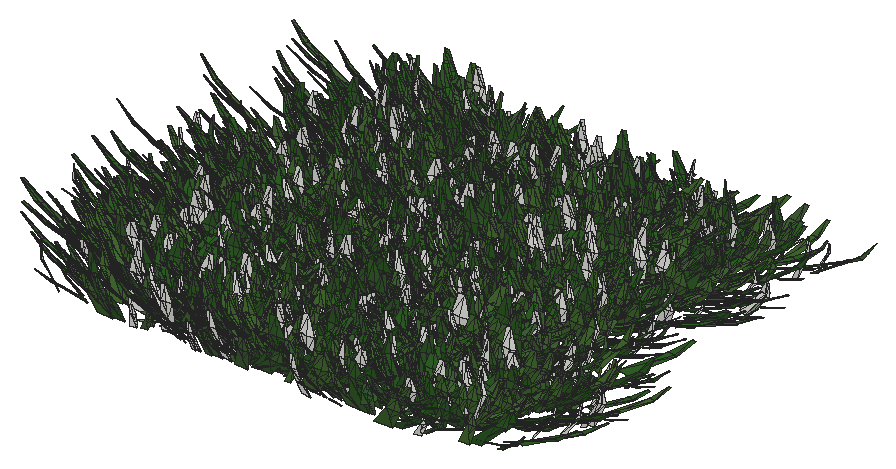
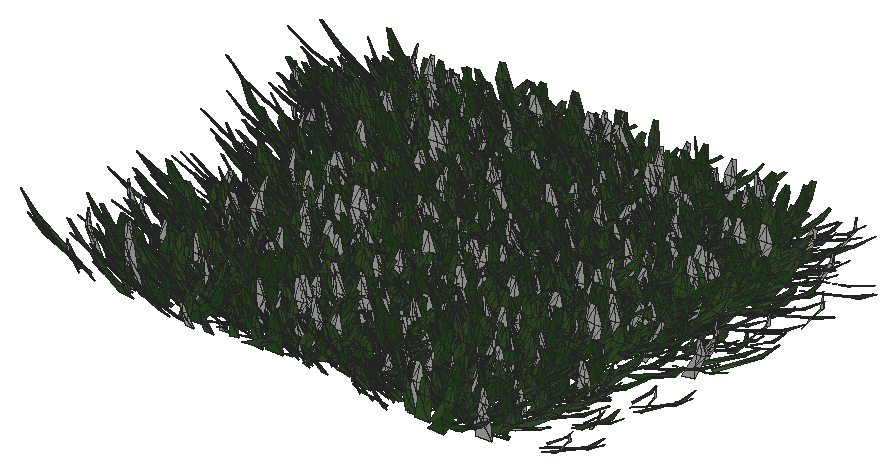
# SketchUp Ruby script. Lengths in inches.
U = 1.inch
M = Sketchup.active_model
def pt(a) = Geom::Point3d.new(a.map { |v| v * U })
def face(e, loops, mat)
  f = e.add_face(loops[0].map { |a| pt(a) })
  loops[1..].each { |l| e.add_face(l.map { |a| pt(a) }).erase! }
  f.material = f.back_material = mat if mat
  f
end
# faces: each face lists its corners as indices into pts; further lists are holes
def faces(e, pts, list, mat = nil) = list.each { |f| face(e, (f[0].is_a?(Array) ? f : [f]).map { |l| l.map { |i| pts[i] } }, mat) }
# xy, xz, yz: faces in a plane at the given z, y or x. An outline is a flat list of corners, or four numbers for a rectangle; further outlines are holes
def ring(l) = l.size == 4 ? [[l[0], l[1]], [l[2], l[1]], [l[2], l[3]], [l[0], l[3]]] : l.each_slice(2).to_a
def flat(e, list, mat, &to3) = list.each { |f| face(e, (f[0].is_a?(Array) ? f : [f]).map { |l| ring(l).map { |u, v| to3.(u, v) } }, mat) }
def xy(e, z, list, mat = nil) = flat(e, list, mat) { |x, y| [x, y, z] }
def xz(e, y, list, mat = nil) = flat(e, list, mat) { |x, z| [x, y, z] }
def yz(e, x, list, mat = nil) = flat(e, list, mat) { |y, z| [x, y, z] }
def lines(e, pts, list) = list.each { |a, b| e.add_line(pt(pts[a]), pt(pts[b])) }
# prism: a flat outline (further loops are holes) pulled along v
def prism(e, loops, v, mat = nil)
  f = face(e, loops, mat); d = Geom::Vector3d.new(v.map { |x| x * U })
  f.pushpull(f.normal.samedirection?(d) ? d.length : -d.length)
end
def box(e, o, s, mat = nil) = prism(e, [[o, [o[0] + s[0], o[1], o[2]], [o[0] + s[0], o[1] + s[1], o[2]], [o[0], o[1] + s[1], o[2]]]], [0, 0, s[2]], mat)
def at(x, y, z, deg = 0) = Geom::Transformation.translation(pt([x, y, z])) * Geom::Transformation.rotation(ORIGIN, Z_AXIS, deg.degrees)
def axes(o, x, y, z) = Geom::Transformation.new([*x, 0, *y, 0, *z, 0, *pt(o).to_a, 1])
def part(name) = M.definitions.add(name)
# library, detail: a bought-in or finely detailed component or shape, given as its bounding box
def library(name, o, s) = part(name).tap { |d| box(d.entities, o, s) }
def detail(e, o, s) = box(e.add_group.entities, o, s)
def put(e, d, t, mat = nil) = e.add_instance(d, t).tap { |i| i.material = mat if mat }
def group(e, t, mat = nil) = e.add_group.tap { |g| g.transformation = t; g.material = mat if mat }.entities
root = M.entities
M.materials.add("Material10").color = [48, 100, 38]
M.materials.add("Material3").color = [68, 110, 58]
M.materials.add("Material4").color = [48, 90, 38]
M.materials.add("Material5").color = [68, 110, 48]
M.materials.add("Material6").color = [48, 90, 48]
M.materials.add("Material7").color = [58, 110, 58]
M.materials.add("Material8").color = [58, 90, 38]
M.materials.add("Material9").color = [68, 100, 58]
c1 = part("grass00")
p = [[-0.6875,0.15,0],[-0.56,0.08,5.52],[-0.04,0.03,2.76],[0.48,-0.02,0],[0.35,-0.02,5.52],[-0.1,-0.14,5.52],
  [-0.12,0.65,8.37],[-0.42,0.65,8.37]]
faces(c1.entities,p,[[0,1,2,3],[3,2,4],[1,5,2],[5,4,2],[1,6,5],[4,5,6],[7,6,1]])
c2 = part("Group16\#1")
put(c2.entities,c1,axes([1.44,-0.61,-0.01],[0.05352,0.12609,0],[-0.10704,0.04543,0.07239],[0.06664,-0.02828,0.11628]),"Material6")
put(c2.entities,c1,axes([0.76,-0.15,-0.01],[0.04676,0.24062,0],[-0.23162,0.04501,0.06642],[0.0652,-0.01267,0.23595]),"Material3")
put(c2.entities,c1,axes([0.79,0.01,-0.01],[-0.00606,0.34651,0],[-0.34381,-0.00602,0.0432],[0.04319,0.00076,0.34386]))
put(c2.entities,c1,axes([1,0.23,-0.01],[-0.07192,0.31144,0],[-0.28722,-0.06632,0.1236],[0.12043,0.02781,0.29478]),"Material5")
put(c2.entities,c1,axes([1.66,0.77,-0.01],[-0.13828,0.29651,0],[-0.21551,-0.1005,0.22471],[0.20365,0.09498,0.23779]),"Material10")
put(c2.entities,c1,axes([0.6875,0.52,-0.01],[-0.18126,0.24051,0],[-0.22746,-0.17142,0.09788],[0.07817,0.05891,0.28481]),"Material5")
put(c2.entities,c1,axes([0.68,0.78,-0.01],[-0.215,0.18688,0],[-0.12385,-0.14248,0.21334],[0.13995,0.16101,0.18878]),"Material3")
put(c2.entities,c1,axes([0.56,1,-0.01],[-0.13756,0.07624,0],[-0.06159,-0.11112,0.0927],[0.04494,0.08108,0.12705]),"Material5")
put(c2.entities,c1,axes([0.2,0.64,-0.01],[-0.23729,0.07254,0],[-0.05711,-0.18681,0.153],[0.04473,0.14632,0.19535]),"Material10")
put(c2.entities,c1,axes([0.0625,0.72,-0.01],[-0.28874,0.02525,0],[-0.02179,-0.24916,0.14647],[0.01276,0.14591,0.25012]),"Material3")
put(c2.entities,c1,axes([-0.08,0.62,-0.01],[-0.34089,-0.04187,0],[0.03255,-0.26504,0.216],[-0.02633,0.21439,0.26703]),"Material10")
put(c2.entities,c1,axes([-0.34,0.98,-0.01],[-0.14314,-0.0493,0],[0.04397,-0.12769,0.06843],[-0.02228,0.0647,0.13505]),"Material10")
put(c2.entities,c1,axes([-0.87,1.45,-0.01],[-0.23488,-0.14114,0],[0.13761,-0.22901,0.06087],[-0.03135,0.05217,0.26717]))
put(c2.entities,c1,axes([-0.72,0.77,-0.01],[-0.14208,-0.13251,0],[0.07209,-0.0773,0.16301],[-0.11118,0.11922,0.1057]),"Material10")
put(c2.entities,c1,axes([-0.62,0.43,-0.01],[-0.14845,-0.21203,0],[0.18654,-0.13061,0.12304],[-0.10079,0.07057,0.22772]),"Material3")
put(c2.entities,c1,axes([-0.68,0.29,-0.01],[-0.13639,-0.32136,0],[0.31723,-0.13464,0.05579],[-0.05136,0.0218,0.34462]),"Material4")
put(c2.entities,c1,axes([-0.64,0.125,-0.01],[-0.0458,-0.23569,0],[0.22124,-0.043,0.08276],[-0.08124,0.01579,0.22538]),"Material7")
put(c2.entities,c1,axes([-1.6,-0.03,-0.01],[0.00576,-0.32897,0],[0.27526,0.00482,0.18018],[-0.18015,-0.00315,0.2753]),"Material5")
put(c2.entities,c1,axes([-1.36,-0.31,-0.01],[0.05718,-0.24765,0],[0.18172,0.04196,0.17267],[-0.16825,-0.03885,0.1865]),"Material10")
put(c2.entities,c1,axes([-1.54,-0.72,-0.01],[0.06537,-0.14017,0],[0.13555,0.06321,0.03939],[-0.0357,-0.01665,0.14956]))
put(c2.entities,c1,axes([-1.19,-0.9,-0.01],[0.09597,-0.12735,0],[0.11214,0.08451,0.07557],[-0.06035,-0.04548,0.14042]),"Material9")
put(c2.entities,c1,axes([-0.47,-0.54,-0.01],[0.11588,-0.10072,0],[0.0618,0.0711,0.12124],[-0.07953,-0.0915,0.0942]))
put(c2.entities,c1,axes([-0.47,-0.84,-0.01],[0.11927,-0.0661,0],[0.06603,0.11913,0.00646],[-0.00313,-0.00565,0.13621]),"Material5")
put(c2.entities,c1,axes([-0.38,-1.24,-0.01],[0.28037,-0.08571,0],[0.0618,0.20215,0.20315],[-0.05939,-0.19428,0.21139]),"Material9")
put(c2.entities,c1,axes([-0.06,-0.66,-0.01],[0.22719,-0.01987,0],[0.01247,0.14255,0.17758],[-0.01547,-0.17691,0.1431]),"Material8")
put(c2.entities,c1,axes([0.11,-0.89,-0.01],[0.14882,0.01828,0],[-0.01058,0.08611,0.12229],[0.01491,-0.12138,0.08676]),"Material6")
put(c2.entities,c1,axes([0.25,-0.72,-0.01],[0.20481,0.07053,0],[-0.06206,0.18022,0.10291],[0.03351,-0.0973,0.1906]),"Material6")
put(c2.entities,c1,axes([0.85,-1.42,-0.01],[0.16481,0.09904,0],[-0.09472,0.15762,0.05616],[0.02893,-0.04814,0.18389]),"Material5")
put(c2.entities,c1,axes([1.01,-1.09,-0.01],[0.21858,0.20385,0],[-0.17495,0.1876,0.15339],[0.10462,-0.11218,0.25652]),"Material10")
put(c2.entities,c1,axes([1.01,-0.71,-0.01],[0.08733,0.12473,0],[-0.06445,0.04512,0.13037],[0.1068,-0.07477,0.07867]),"Material6")
c3 = part("Group15\#1")
put(c3.entities,c2,at(0,0,0))
c4 = part("3darcstudiotree_grass00\#1")
put(c4.entities,c3,at(0,0,0))
put(root,c4,axes([993.08,950.1,0],[-3.70141,-0.8816,0],[3.55908,-0.93393,-0.03405],[0.10659,-0.02797,1.46358]))
put(root,c4,axes([990.92,944.4375,0],[1.53914,1.0513,0],[-4.39566,0.40221,-0.03042],[-0.15696,0.01436,1.60735]))
put(root,c4,axes([991.4,954.42,0],[4.38638,0.43915,0],[-1.65781,1.03492,-0.05201],[-0.12203,0.07618,1.75905]))
put(root,c4,axes([992.45,966.72,0],[3.5333,-0.35922,0],[1.45173,0.89244,-0.02601],[0.05982,0.03677,1.4702]))
put(root,c4,axes([992.18,962.12,0],[4.6185,-0.19049,0],[0.64707,0.98053,-0.03976],[0.0459,0.06956,1.7619]))
put(root,c4,axes([992.69,939.44,0],[-0.10897,1.07036,0],[-4.26555,-0.02714,-0.03168],[-0.19713,-0.00125,1.66016]))
put(root,c4,axes([993.28,951.7,0],[3.42773,-0.49366,0],[2.33187,1.01196,-0.00508],[0.01362,0.00591,1.56982]))
put(root,c4,axes([992.8,948.71,0],[1.88253,1.20428,0],[-4.05103,0.39579,-0.05423],[-0.25457,0.02487,1.37014]))
put(root,c4,axes([994.36,945.55,0],[1.67023,-1.19421,0],[4.03376,0.3526,-0.01723],[0.08743,0.00764,1.43549]))
put(root,c4,axes([993.875,938.22,0],[-2.65738,1.09384,0],[-4.1127,-0.62446,-0.06137],[-0.25477,-0.03868,1.46064]))
put(root,c4,axes([993.53,942.125,0],[3.93411,-0.32217,0],[1.27665,0.97436,-0.03684],[0.07239,0.05525,1.61813]))
put(root,c4,axes([993.77,971.11,0],[4.66298,-0.3319,0],[1.18544,1.04091,-0.0361],[0.05479,0.04811,1.4995]))
put(root,c4,axes([994.79,946.65,0],[-3.31735,0.93033,0],[-2.98242,-0.66466,-0.02096],[-0.10528,-0.02346,1.6805]))
put(root,c4,axes([994.64,957.16,0],[-1.67728,0.97063,0],[-4.3061,-0.46507,-0.05011],[-0.26514,-0.02864,1.6899]))
put(root,c4,axes([995.03,955.6,0],[-2.6954,0.74968,0],[-3.20953,-0.72123,-0.05045],[-0.20663,-0.04643,1.48531]))
put(root,c4,axes([994.5,965.08,0],[0.74763,1.2665,0],[-3.58863,0.1324,-0.00575],[-0.0331,0.00122,1.31904]))
put(root,c4,axes([994.71,933.67,0],[0.50371,0.92792,0],[-3.91618,0.13287,-0.02967],[-0.18729,0.00635,1.57371]))
put(root,c4,axes([996.82,964.2,0],[-3.39734,-0.81214,0],[3.21264,-0.83994,-0.00934],[0.03489,-0.00912,1.57129]))
put(root,c4,axes([994.63,952.85,0],[2.9171,1.0312,0],[-3.90665,0.69071,-0.03132],[-0.15312,0.02707,1.7905]))
put(root,c4,axes([997.03,966.61,0],[-3.12061,-0.47334,0],[2.372,-0.97738,-0.04577],[0.16283,-0.06709,1.96036]))
put(root,c4,axes([997.5625,964.73,0],[-4.51264,-0.18826,0],[0.71719,-1.07444,-0.03361],[0.0313,-0.04689,1.54092]))
put(root,c4,axes([997.93,954.32,0],[-1.81184,-1.16372,0],[3.89157,-0.37868,-0.00938],[0.0544,-0.00529,1.62403]))
put(root,c4,axes([998.05,947.21,0],[-2.30449,-0.91323,0],[3.99186,-0.62958,-0.04882],[0.19366,-0.03054,1.38366]))
put(root,c4,axes([997.91,958.86,0],[-3.97113,-0.2451,0],[1.12308,-1.13729,-0.03453],[0.04096,-0.04148,1.44935]))
put(root,c4,axes([996.7,962.68,0],[0.9039,1.10782,0],[-3.7396,0.1907,-0.03877],[-0.30879,0.01575,1.93915]))
put(root,c4,axes([997.12,943.48,0],[4.31287,-0.5541,0],[2.34742,1.14195,-0.04443],[0.08836,0.04298,1.39643]))
put(root,c4,axes([998.5,949.51,0],[-2.23159,-0.76023,0],[4.05726,-0.74436,-0.05528],[0.25257,-0.04634,1.78248]))
put(root,c4,axes([998.52,948.84,0],[-4.02658,-0.46054,0],[1.58874,-0.86816,-0.02741],[0.08919,-0.04874,1.86713]))
put(root,c4,axes([996.73,951.7,0],[4.23303,0.24806,0],[-0.88984,0.94903,-0.007],[-0.01026,0.01094,1.56436]))
put(root,c4,axes([997.01,956.24,0],[0.42645,1.00239,0],[-4.44972,0.11832,-0.05804],[-0.28832,0.00767,1.39706]))
put(root,c4,axes([997,970.93,0],[3.77106,0.1861,0],[-0.77685,0.98386,-0.02055],[-0.02979,0.03773,1.87683]))
put(root,c4,axes([998.93,940.92,0],[-3.30832,-0.44964,0],[1.76308,-0.81076,-0.02167],[0.05991,-0.02755,1.33527]))
put(root,c4,axes([998.79,960.9375,0],[-4.45965,0.06137,0],[-0.23794,-1.08073,-0.00024],[-0.00009,-0.00042,1.85086]))
put(root,c4,axes([998.5,935.0625,0],[-3.86065,0.46316,0],[-1.72487,-0.89859,-0.02803],[-0.09373,-0.04883,1.92571]))
put(root,c4,axes([997.53,972.55,0],[0.27692,1.06146,0],[-3.97037,0.06474,-0.03468],[-0.23973,0.00391,1.72254]))
put(root,c4,axes([998.02,945.57,0],[4.229,-0.39119,0],[1.33455,0.9017,-0.04569],[0.11742,0.07934,1.78027]))
put(root,c4,axes([999.43,969.71,0],[-4.92673,0.10496,0],[-0.34343,-1.00748,-0.04489],[-0.0281,-0.08244,1.86365]))
put(root,c4,axes([998.88,942.19,0],[2.71553,-0.59411,0],[3.06461,0.87548,-0.0129],[0.0406,0.0116,1.39029]))
put(root,c4,axes([998.58,953.56,0],[4.13058,-0.51477,0],[2.24071,1.12373,-0.00236],[0.00471,0.00236,1.40454]))
put(root,c4,axes([999.89,968.64,0],[-4.32782,-0.07969,0],[0.34618,-1.17501,-0.00991],[0.00419,-0.01422,1.69565]))
put(root,c4,axes([998.53,937.6875,0],[4.87575,-0.07031,0],[0.2378,1.03062,-0.03809],[0.01526,0.06615,1.79573]))
put(root,c4,axes([999,936.71,0],[4.34695,-0.61956,0],[2.03841,0.89387,-0.05304],[0.19031,0.08345,1.86337]))
put(root,c4,axes([1000.55,939.22,0],[-0.06657,-0.97228,0],[3.61389,-0.01547,-0.01279],[0.09363,-0.0004,1.65408]))
put(root,c4,axes([1000.48,957.67,0],[-0.52118,1.08575,0],[-3.57431,-0.10723,-0.01529],[-0.11274,-0.00338,1.67142]))
put(root,c4,axes([1002.68,939.83,0],[-0.33547,-0.93865,0],[4.62281,-0.10326,-0.01785],[0.11677,-0.00261,1.90542]))
put(root,c4,axes([1002.77,940.375,0],[0.01005,-1.20258,0],[4.19815,0.00219,-0.00952],[0.05269,0.00003,1.45276]))
put(root,c4,axes([1003.34,957.1,0],[-4.31518,-0.12187,0],[0.57213,-1.26614,-0.03054],[0.01977,-0.04376,1.83699]))
put(root,c4,axes([1003.46,962.26,0],[-3.97014,0.26009,0],[-1.01896,-0.97211,-0.00505],[-0.00887,-0.00846,1.74136]))
put(root,c4,axes([1002.71,951.42,0],[3.84845,-0.37536,0],[1.314,0.842,-0.03886],[0.09501,0.06088,1.52001]))
put(root,c4,axes([1004.52,971.2,0],[-3.84586,-0.50053,0],[1.98165,-0.95164,-0.02288],[0.06035,-0.02898,1.53217]))
put(root,c4,axes([1004.54,956.28,0],[1.58704,-0.95278,0],[3.80003,0.3956,-0.04485],[0.25602,0.02665,1.59096]))
put(root,c4,axes([1003.58,937.61,0],[0.72703,0.98679,0],[-4.37824,0.20161,-0.0472],[-0.24448,0.01126,1.46547]))
put(root,c4,axes([1003.69,953.25,0],[2.85718,1.03717,0],[-3.15985,0.54404,-0.04649],[-0.2079,0.0358,1.30192]))
put(root,c4,axes([1003.82,945.07,0],[4.19495,0.19536,0],[-0.69064,0.92689,-0.03922],[-0.04451,0.05974,1.46066]))
put(root,c4,axes([1004.42,955.03,0],[3.26699,-0.39523,0],[1.71248,0.88472,-0.0104],[0.02647,0.01367,1.43546]))
put(root,c4,axes([1003.76,963.12,0],[0.48352,1.11677,0],[-5.03625,0.13628,-0.03135],[-0.15085,0.00408,1.53244]))
put(root,c4,axes([1004.44,965.01,0],[4.15736,-0.22719,0],[0.90665,1.03692,-0.02018],[0.02441,0.02792,1.50307]))
put(root,c4,axes([1006.59,948.11,0],[-2.6745,-0.8431,0],[3.5822,-0.71022,-0.01126],[0.04091,-0.00811,1.32461]))
put(root,c4,axes([1006.23,944.43,0],[-3.71389,-0.2193,0],[0.91243,-0.96576,-0.01801],[0.02228,-0.02358,1.33554]))
put(root,c4,axes([1006.1,942.16,0],[-1.37594,-0.94184,0],[3.46555,-0.31643,-0.03784],[0.25579,-0.02336,1.65933]))
put(root,c4,axes([1006.53,967.89,0],[-0.30959,-1.20063,0],[5.07298,-0.08176,-0.03565],[0.17141,-0.00276,1.53082]))
put(root,c4,axes([1006.7,949.87,0],[-5.13737,-0.16678,0],[0.63051,-1.21389,-0.02421],[0.01691,-0.03256,1.66024]))
put(root,c4,axes([1005.71,966.95,0],[2.61832,-0.717,0],[3.31257,0.75605,-0.05494],[0.2657,0.06064,1.83588]))
put(root,c4,axes([1005.74,936.28,0],[4.35597,0.12735,0],[-0.44802,0.95775,-0.0104],[-0.00937,0.02004,1.87036]))
put(root,c4,axes([1006.67,961.1,0],[2.88619,-0.79207,0],[3.8321,0.87272,-0.04921],[0.18723,0.04264,1.66765]))
put(root,c4,axes([1006.53,959.3,0],[-2.47521,0.9479,0],[-4.1372,-0.67521,-0.02867],[-0.13874,-0.02264,1.78429]))
put(root,c4,axes([1006.01,933.64,0],[3.15699,0.44702,0],[-1.9309,0.8523,-0.02459],[-0.09443,0.04168,1.90817]))
put(root,c4,axes([1006.77,947.3,0],[4.16611,-0.6608,0],[2.43007,0.95755,-0.04672],[0.16308,0.06426,1.84728]))
put(root,c4,axes([1006.1,934.39,0],[3.70483,0.88926,0],[-3.42802,0.89261,-0.04664],[-0.18584,0.04839,1.77978]))
put(root,c4,axes([1006.75,969.4,0],[1.28426,1.18436,0],[-4.11752,0.27905,-0.02312],[-0.12583,0.00853,1.50331]))
put(root,c4,axes([1009.34,949.63,0],[2.28346,-0.77469,0],[3.44717,0.63505,-0.04551],[0.22499,0.04145,1.64335]))
put(root,c4,axes([1009.38,945.4,0],[-3.11661,0.81451,0],[-3.35485,-0.80231,-0.01205],[-0.05625,-0.01345,1.87482]))
put(root,c4,axes([1010.51,938.44,0],[-4.56857,-0.03056,0],[0.12408,-1.1593,-0.01377],[0.0021,-0.01961,1.65227]))
put(root,c4,axes([1010.05,955.05,0],[-3.49798,0.58152,0],[-2.29705,-0.86358,-0.00165],[-0.005,-0.00188,1.42237]))
put(root,c4,axes([1011.08,942.18,0],[-3.54461,-0.42652,0],[2.22844,-1.15748,-0.00367],[0.00795,-0.00413,1.60507]))
put(root,c4,axes([1010.65,936.26,0],[0.72449,-1.28293,0],[4.25597,0.15021,-0.01886],[0.1212,0.00428,1.74385]))
put(root,c4,axes([1009.57,952.7,0],[4.06118,0.1391,0],[-0.5324,0.97148,-0.00884],[-0.00926,0.01689,1.89082]))
put(root,c4,axes([1009.73,970.2,0],[3.80962,0.48399,0],[-2.27163,1.11755,-0.02666],[-0.05719,0.02813,1.48409]))
put(root,c4,axes([1010.35,934.4,0],[-1.84818,0.79503,0],[-4.49204,-0.65265,-0.02835],[-0.13063,-0.01898,1.73088]))
put(root,c4,axes([1011.93,965.32,0],[-4.49893,-0.43837,0],[1.53995,-0.98776,-0.03755],[0.08017,-0.05142,1.55797]))
put(root,c4,axes([1010.35,963.24,0],[4.7752,0.14497,0],[-0.46713,0.96169,-0.01966],[-0.01749,0.036,1.78732]))
put(root,c4,axes([1010.83,957.28,0],[-1.92575,0.83965,0],[-4.05155,-0.58077,-0.01882],[-0.10891,-0.01561,1.94745]))
put(root,c4,axes([1012.52,962.59,0],[-1.58063,-0.88051,0],[4.29272,-0.48163,-0.01184],[0.05795,-0.0065,1.57815]))
put(root,c4,axes([1012.26,966.58,0],[-0.4942,-0.9258,0],[4.62783,-0.1544,-0.03174],[0.19168,-0.0064,1.77768]))
put(root,c4,axes([1011.22,940.77,0],[4.19202,-0.62373,0],[2.32182,0.97529,-0.02674],[0.0725,0.03045,1.50406]))
put(root,c4,axes([1012.4,968.29,0],[-2.7199,-1.09643,0],[3.70626,-0.57463,-0.05324],[0.3066,-0.04754,1.84703]))
put(root,c4,axes([1012.27,951.14,0],[-4.05366,0.12739,0],[-0.60907,-1.21134,-0.04842],[-0.03855,-0.07666,1.94818]))
put(root,c4,axes([1011.39,948.84,0],[5.04215,0.13014,0],[-0.5216,1.26309,-0.06196],[-0.03085,0.07472,1.53928]))
put(root,c4,axes([1011.625,939.08,0],[4.01222,0.17516,0],[-0.82819,1.18564,-0.04039],[-0.03228,0.04621,1.39779]))
put(root,c4,axes([1011.9,947.32,0],[3.70391,0.67264,0],[-2.69019,0.92586,-0.05492],[-0.18493,0.06364,1.63919]))
put(root,c4,axes([1013.2,970.81,0],[-3.854,0.71401,0],[-2.71385,-0.91553,-0.03727],[-0.14645,-0.04941,1.88005]))
put(root,c4,axes([1012.6,956.61,0],[3.9405,-0.83524,0],[2.79845,0.82516,-0.04452],[0.20818,0.06139,1.95574]))
put(root,c4,axes([1011.73,959.53,0],[2.7963,0.73348,0],[-3.70563,0.88296,-0.0237],[-0.07242,0.01726,1.35093]))
put(root,c4,axes([1012.88,944.37,0],[3.48051,0.83109,0],[-2.69675,0.70586,-0.00574],[-0.02303,0.00603,1.41814]))
put(root,c4,axes([1013.1,960.93,0],[1.55604,0.87534,0],[-4.29389,0.47706,-0.00487],[-0.02529,0.00281,1.66894]))
put(root,c4,axes([1016.02,936.34,0],[-4.60072,-0.1914,0],[0.66397,-0.99747,-0.03971],[0.03807,-0.05719,1.4765]))
put(root,c4,axes([1015.3,968.43,0],[-2.80563,0.59342,0],[-3.19145,-0.94305,-0.04396],[-0.1676,-0.04953,1.82298]))
put(root,c4,axes([1015.375,969.18,0],[-3.36424,0.91814,0],[-3.26593,-0.74794,-0.02313],[-0.11922,-0.0273,1.93523]))
put(root,c4,axes([1015.37,941.01,0],[3.31986,-0.90832,0],[2.95695,0.67547,-0.04297],[0.18756,0.04285,1.48019]))
put(root,c4,axes([1015.27,942.84,0],[4.45796,-0.3025,0],[1.23547,1.13796,-0.0215],[0.03263,0.03006,1.70776]))
put(root,c4,axes([1015.01,960.45,0],[1.59432,0.97436,0],[-4.70635,0.4813,-0.06498],[-0.3656,0.03739,1.93183]))
put(root,c4,axes([1015.625,950.4,0],[4.36905,-0.5157,0],[1.63569,0.86611,-0.01833],[0.04371,0.02315,1.33779]))
put(root,c4,axes([1015.54,951.82,0],[-2.09066,0.8963,0],[-4.13643,-0.60302,-0.00159],[-0.00743,-0.00108,1.61385]))
put(root,c4,axes([1015.46,964.9,0],[3.77784,0.09096,0],[-0.38847,1.00844,-0.03978],[-0.02973,0.07718,1.9745]))
put(root,c4,axes([1016.16,957.25,0],[4.39293,-0.39638,0],[1.51129,1.04681,-0.00463],[0.01009,0.00699,1.7876]))
put(root,c4,axes([1017.8,935.34,0],[-2.80912,-0.5814,0],[2.98833,-0.9024,-0.02106],[0.0666,-0.02011,1.45262]))
put(root,c4,axes([1015.59,947.99,0],[1.32804,0.89243,0],[-4.56048,0.42416,-0.01219],[-0.04894,0.00455,1.30286]))
put(root,c4,axes([1016.95,943.6,0],[-3.32952,0.73934,0],[-2.566,-0.72222,-0.02123],[-0.07998,-0.02251,1.37003]))
put(root,c4,axes([1017.18,947.54,0],[1.3987,-1.16529,0],[3.94932,0.29627,-0.0465],[0.25173,0.01888,1.45674]))
put(root,c4,axes([1016.17,939.12,0],[4.48384,-0.0442,0],[0.16896,1.07134,-0.03451],[0.00949,0.06019,1.8714]))
put(root,c4,axes([1018.1,971.47,0],[-2.9743,-0.97046,0],[3.84774,-0.73704,-0.04805],[0.20355,-0.03899,1.61679]))
put(root,c4,axes([1016.11,937.74,0],[3.76585,0.33599,0],[-1.61193,1.12919,-0.03925],[-0.05722,0.04008,1.29995]))
put(root,c4,axes([1017.62,966.16,0],[1.03504,-1.15768,0],[4.4608,0.24927,-0.0396],[0.20091,0.01123,1.48525]))
put(root,c4,axes([1017.12,959.42,0],[3.13436,-0.48515,0],[2.36256,0.95397,-0.03178],[0.09873,0.03987,1.65559]))
put(root,c4,axes([1016.8125,963.28,0],[2.27275,0.69978,0],[-3.25332,0.66039,-0.04172],[-0.2207,0.0448,1.78477]))
put(root,c4,axes([1018.49,961.87,0],[0.03995,-0.91638,0],[3.85114,0.01049,-0.01263],[0.08929,0.00024,1.70174]))
put(root,c4,axes([1018.74,945.21,0],[-0.0743,-1.09346,0],[5.15443,-0.02189,-0.0635],[0.38021,-0.00161,1.92948]))
put(root,c4,axes([1018.35,954.79,0],[-0.87822,1.20362,0],[-5.10038,-0.23259,-0.02378],[-0.14141,-0.00645,1.95907]))
put(root,c4,axes([1018.68,933.62,0],[-1.6227,0.88053,0],[-4.355,-0.50161,-0.00587],[-0.0262,-0.00302,1.47291]))
put(root,c4,axes([1018.72,955.59,0],[4.89448,0.02106,0],[-0.07768,1.1284,-0.04862],[-0.00413,0.05993,1.39123]))
put(root,c4,axes([1019.23,952.88,0],[3.93844,-0.46233,0],[1.56764,0.83463,-0.03796],[0.10707,0.05701,1.52986]))
put(root,c4,axes([1021.36,940.96,0],[-4.19523,0.01101,0],[-0.04384,-1.04387,-0.01485],[-0.00097,-0.02314,1.62647]))
put(root,c4,axes([1021.25,960.9,0],[2.74476,-0.63144,0],[3.24378,0.88126,-0.00074],[0.00283,0.00077,1.68668]))
put(root,c4,axes([1021.92,950.5,0],[-1.38491,-0.87134,0],[4.17889,-0.41512,-0.04918],[0.21859,-0.02171,1.34418]))
put(root,c4,axes([1021.29,956.09,0],[-2.83927,0.94701,0],[-3.75848,-0.70428,-0.01976],[-0.09358,-0.01754,1.7373]))
put(root,c4,axes([1021.03,957.5,0],[4.64321,-0.10228,0],[0.43492,1.23399,-0.00682],[0.00288,0.00819,1.49182]))
put(root,c4,axes([1022.4,951.83,0],[0.60172,-0.90687,0],[4.84176,0.20079,-0.06063],[0.30013,0.01245,1.53907]))
put(root,c4,axes([1021.15,966.8,0],[4.59228,0.4506,0],[-1.57539,1.00348,-0.00074],[-0.00157,0.001,1.56313]))
put(root,c4,axes([1023.3,958.86,0],[-4.3908,-0.21331,0],[0.95341,-1.22655,-0.00093],[0.00081,-0.00104,1.42207]))
put(root,c4,axes([1023.45,964.87,0],[-2.23417,-0.72587,0],[3.44566,-0.66284,-0.03027],[0.1304,-0.02509,1.47708]))
put(root,c4,axes([1021.53,954.76,0],[0.72512,1.17526,0],[-3.95245,0.15241,-0.0058],[-0.04155,0.0016,1.813]))
put(root,c4,axes([1023.16,943.56,0],[1.59637,-0.98272,0],[4.08137,0.41437,-0.04502],[0.2819,0.02862,1.86083]))
put(root,c4,axes([1022.8,936.9,0],[3.44919,-0.8389,0],[2.51647,0.64667,-0.01443],[0.08324,0.02139,1.86565]))
put(root,c4,axes([1024.07,946.57,0],[-4.3854,-0.36655,0],[1.15878,-0.86648,-0.00172],[0.00341,-0.00255,1.42531]))
put(root,c4,axes([1024.18,937.46,0],[-1.10015,-1.07569,0],[4.31851,-0.27604,-0.04783],[0.26751,-0.0171,1.6084]))
put(root,c4,axes([1024.53,963.45,0],[-2.44496,-0.90858,0],[3.92777,-0.66059,-0.0439],[0.19033,-0.03201,1.54604]))
put(root,c4,axes([1022.54,953.47,0],[3.01882,0.54467,0],[-2.85178,0.98787,-0.01696],[-0.0599,0.02075,1.8379]))
put(root,c4,axes([1022.78,945.96,0],[1.72651,0.80182,0],[-4.15188,0.55875,-0.00648],[-0.03257,0.00438,1.68262]))
put(root,c4,axes([1024.76,971.45,0],[-4.67562,0.03677,0],[-0.12525,-0.99545,-0.03177],[-0.00796,-0.06328,1.98473]))
put(root,c4,axes([1023,967.87,0],[3.74443,0.79231,0],[-2.92784,0.86481,-0.04954],[-0.20172,0.05958,1.78537]))
put(root,c4,axes([1025.29,938.84,0],[-0.41267,-0.99142,0],[5.06334,-0.13172,-0.00351],[0.0163,-0.00042,1.48465]))
put(root,c4,axes([1023.33,935.42,0],[4.97186,0.0872,0],[-0.33381,1.18949,-0.05051],[-0.02266,0.08074,1.91076]))
put(root,c4,axes([1025.3,969.89,0],[-2.51888,-0.8121,0],[2.88545,-0.55936,-0.0081],[0.05261,-0.0102,1.87526]))
put(root,c4,axes([1024.9,962.09,0],[0.49939,-1.21812,0],[4.94049,0.12659,-0.06373],[0.30684,0.00786,1.50237]))
put(root,c4,axes([1024.86,941.89,0],[1.78182,-0.82345,0],[4.25701,0.57572,-0.03985],[0.17401,0.02353,1.5017]))
put(root,c4,axes([1024.38,948.32,0],[4.57283,0.48925,0],[-2.0405,1.19199,-0.06274],[-0.14636,0.0855,1.92197]))
put(root,c4,axes([1027.01,942.97,0],[-4.16521,-0.5533,0],[2.06422,-0.97121,-0.03648],[0.11162,-0.05251,1.79293]))
put(root,c4,axes([1026.9375,941.37,0],[-2.37661,-1.01523,0],[3.11528,-0.4558,-0.0221],[0.1541,-0.02255,1.82262]))
